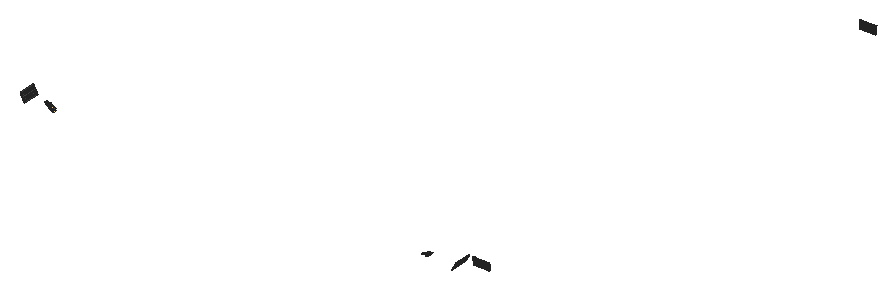
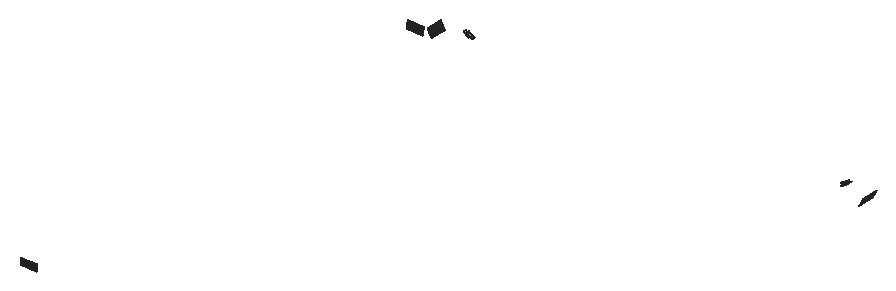
# SketchUp Ruby script. Lengths in inches.
U = 1.inch
M = Sketchup.active_model
def pt(a) = Geom::Point3d.new(a.map { |v| v * U })
def face(e, loops, mat)
  f = e.add_face(loops[0].map { |a| pt(a) })
  loops[1..].each { |l| e.add_face(l.map { |a| pt(a) }).erase! }
  f.material = f.back_material = mat if mat
  f
end
# faces: each face lists its corners as indices into pts; further lists are holes
def faces(e, pts, list, mat = nil) = list.each { |f| face(e, (f[0].is_a?(Array) ? f : [f]).map { |l| l.map { |i| pts[i] } }, mat) }
# xy, xz, yz: faces in a plane at the given z, y or x. An outline is a flat list of corners, or four numbers for a rectangle; further outlines are holes
def ring(l) = l.size == 4 ? [[l[0], l[1]], [l[2], l[1]], [l[2], l[3]], [l[0], l[3]]] : l.each_slice(2).to_a
def flat(e, list, mat, &to3) = list.each { |f| face(e, (f[0].is_a?(Array) ? f : [f]).map { |l| ring(l).map { |u, v| to3.(u, v) } }, mat) }
def xy(e, z, list, mat = nil) = flat(e, list, mat) { |x, y| [x, y, z] }
def xz(e, y, list, mat = nil) = flat(e, list, mat) { |x, z| [x, y, z] }
def yz(e, x, list, mat = nil) = flat(e, list, mat) { |y, z| [x, y, z] }
def lines(e, pts, list) = list.each { |a, b| e.add_line(pt(pts[a]), pt(pts[b])) }
# prism: a flat outline (further loops are holes) pulled along v
def prism(e, loops, v, mat = nil)
  f = face(e, loops, mat); d = Geom::Vector3d.new(v.map { |x| x * U })
  f.pushpull(f.normal.samedirection?(d) ? d.length : -d.length)
end
def box(e, o, s, mat = nil) = prism(e, [[o, [o[0] + s[0], o[1], o[2]], [o[0] + s[0], o[1] + s[1], o[2]], [o[0], o[1] + s[1], o[2]]]], [0, 0, s[2]], mat)
def at(x, y, z, deg = 0) = Geom::Transformation.translation(pt([x, y, z])) * Geom::Transformation.rotation(ORIGIN, Z_AXIS, deg.degrees)
def axes(o, x, y, z) = Geom::Transformation.new([*x, 0, *y, 0, *z, 0, *pt(o).to_a, 1])
def part(name) = M.definitions.add(name)
# library, detail: a bought-in or finely detailed component or shape, given as its bounding box
def library(name, o, s) = part(name).tap { |d| box(d.entities, o, s) }
def detail(e, o, s) = box(e.add_group.entities, o, s)
def put(e, d, t, mat = nil) = e.add_instance(d, t).tap { |i| i.material = mat if mat }
def group(e, t, mat = nil) = e.add_group.tap { |g| g.transformation = t; g.material = mat if mat }.entities
root = M.entities
M.materials.add("1432 AP 8245 TAR ROAD").color = [71, 72, 75]
M.materials.add("Outer Light").color = [251, 217, 152]
p = [[248.91,107.37,172.03],[249.07,107.37,171.79],[249.07,95.37,171.79],[248.91,95.37,172.03],[566.93,107.37,171.79],[567.09,107.37,172.03],
  [567.09,95.37,172.03],[566.93,95.37,171.79],[573,108.18,172.22],[573,108.24,171.9375],[585,108.24,171.9375],[585,108.18,172.22],
  [573,466.5,171.9375],[573,466.5625,172.22],[585,466.5625,172.22],[585,466.5,171.9375],[248.76,107.37,172.26],[248.76,95.37,172.26],
  [567.24,107.37,172.26],[567.24,95.37,172.26],[573,108.12,172.49],[585,108.12,172.49],[573,466.62,172.49],[585,466.62,172.49],
  [248.6,107.37,172.5],[248.6,95.37,172.5],[567.4,107.37,172.5],[567.4,95.37,172.5],[248.45,107.37,172.74],[248.45,95.37,172.74],
  [567.55,107.37,172.74],[567.55,95.37,172.74],[573,108.0625,172.77],[585,108.0625,172.77],[573,466.68,172.77],[585,466.68,172.77],
  [248.3,107.37,172.98],[248.3,95.37,172.98],[567.7,107.37,172.98],[567.7,95.37,172.98],[573,108.01,173.05],[585,108.01,173.05],
  [573,466.73,173.05],[585,466.73,173.05],[270.86,96.87,172.98],[271.01,96.87,172.91],[271.01,95.37,172.91],[270.86,95.37,172.98],
  [248.16,107.37,173.22],[248.16,95.37,173.22],[270.5625,96.87,173.11],[270.71,96.87,173.04],[270.71,95.37,173.04],[270.5625,95.37,173.11],
  [567.84,107.37,173.22],[567.84,95.37,173.22],[573,107.96,173.32],[585,107.96,173.32],[573,466.78,173.32],[585,466.78,173.32],
  [270.42,96.87,173.18],[270.42,95.37,173.18],[248.01,107.37,173.47],[248.01,95.37,173.47],[270.125,96.87,173.3125],[270.27,96.87,173.24],
  [270.27,95.37,173.24],[270.125,95.37,173.3125],[567.99,107.37,173.47],[567.99,95.37,173.47],[269.98,96.87,173.38],[269.98,95.37,173.38],
  [573,107.91,173.6],[585,107.91,173.6],[573,466.83,173.6],[585,466.83,173.6],[269.84,96.87,173.45],[269.84,95.37,173.45],
  [247.87,107.37,173.71],[247.87,95.37,173.71],[269.55,96.87,173.6],[269.69,96.87,173.53],[269.69,95.37,173.53],[269.55,95.37,173.6],
  [568.13,107.37,173.71],[568.13,95.37,173.71],[269.41,96.87,173.67],[269.41,95.37,173.67],[573,107.86,173.88],[585,107.86,173.88],
  [573,466.88,173.88],[585,466.88,173.88],[247.73,107.37,173.96],[247.73,95.37,173.96],[269.27,96.87,173.75],[269.27,95.37,173.75],
  [568.27,107.37,173.96],[568.27,95.37,173.96],[268.98,96.87,173.91],[269.125,96.87,173.83],[269.125,95.37,173.83],[268.98,95.37,173.91],
  [268.84,96.87,173.99],[268.84,95.37,173.99],[573,107.8125,174.16],[585,107.8125,174.16],[573,466.93,174.16],[585,466.93,174.16],
  [247.59,107.37,174.2],[247.59,95.37,174.2],[268.7,96.87,174.07],[268.7,95.37,174.07],[568.41,107.37,174.2],[568.41,95.37,174.2],
  [268.43,96.87,174.23],[268.56,96.87,174.15],[268.56,95.37,174.15],[268.43,95.37,174.23],[247.45,107.37,174.45],[247.45,95.37,174.45],
  [268.29,96.87,174.3125],[268.29,95.37,174.3125],[568.55,107.37,174.45],[568.55,95.37,174.45],[573,107.77,174.44],[585,107.77,174.44],
  [573,466.97,174.44],[585,466.97,174.44],[268.15,96.87,174.4],[268.15,95.37,174.4],[247.32,107.37,174.7],[247.32,95.37,174.7],
  [268.02,95.37,174.48],[268.15,95.37,174.4],[268.15,96.87,174.4],[268.02,96.87,174.48],[268.02,96.87,174.48],[268.02,95.37,174.48],
  [271.32,95.37,174.41],[271.18,95.37,174.48],[271.18,96.87,174.48],[271.32,96.87,174.41],[271.32,96.87,174.41],[271.18,96.87,174.48],
  [271.18,95.37,174.48],[271.32,95.37,174.41],[544.68,96.87,174.41],[544.55,96.87,174.35],[544.55,95.37,174.35],[544.68,95.37,174.41],
  [544.82,96.87,174.48],[544.82,95.37,174.48],[544.82,95.37,174.48],[544.68,95.37,174.41],[544.68,96.87,174.41],[544.82,96.87,174.48],
  [547.85,95.37,174.4],[547.98,95.37,174.48],[547.98,96.87,174.48],[547.85,96.87,174.4],[547.85,96.87,174.4],[547.98,96.87,174.48],
  [547.98,95.37,174.48],[547.85,95.37,174.4],[568.68,107.37,174.7],[568.68,95.37,174.7],[573,107.73,174.72],[585,107.73,174.72],
  [573,467.01,174.72],[585,467.01,174.72],[267.88,95.37,174.57],[267.88,96.87,174.57],[267.88,96.87,174.57],[267.88,95.37,174.57],
  [271.05,95.37,174.54],[270.91,95.37,174.6],[270.91,96.87,174.6],[271.05,96.87,174.54],[271.05,96.87,174.54],[270.91,96.87,174.6],
  [270.91,95.37,174.6],[271.05,95.37,174.54],[544.95,96.87,174.54],[544.95,95.37,174.54],[544.95,95.37,174.54],[544.95,96.87,174.54],
  [545.09,96.87,174.6],[545.09,95.37,174.6],[545.09,95.37,174.6],[545.09,96.87,174.6],[548.12,95.37,174.57],[548.12,96.87,174.57],
  [548.12,96.87,174.57],[548.12,95.37,174.57],[267.75,95.37,174.66],[267.75,96.87,174.66],[267.75,96.87,174.66],[267.75,95.37,174.66],
  [270.78,95.37,174.66],[270.78,96.87,174.66],[270.78,96.87,174.66],[270.78,95.37,174.66],[545.22,96.87,174.66],[545.22,95.37,174.66],
  [545.22,95.37,174.66],[545.22,96.87,174.66],[548.25,95.37,174.66],[548.25,96.87,174.66],[548.25,96.87,174.66],[548.25,95.37,174.66],
  [247.18,107.37,174.95],[247.18,95.37,174.95],[267.48,95.37,174.84],[267.61,95.37,174.75],[267.61,96.87,174.75],[267.48,96.87,174.84],
  [267.48,96.87,174.84],[267.61,96.87,174.75],[267.61,95.37,174.75],[267.48,95.37,174.84],[270.64,95.37,174.73],[270.51,95.37,174.8],
  [270.51,96.87,174.8],[270.64,96.87,174.73],[270.64,96.87,174.73],[270.51,96.87,174.8],[270.51,95.37,174.8],[270.64,95.37,174.73],
  [545.36,96.87,174.73],[545.36,95.37,174.73],[545.36,95.37,174.73],[545.36,96.87,174.73],[545.49,96.87,174.8],[545.49,95.37,174.8],
  [545.49,95.37,174.8],[545.49,96.87,174.8],[548.39,95.37,174.75],[548.39,96.87,174.75],[548.39,96.87,174.75],[548.39,95.37,174.75],
  [548.52,95.37,174.84],[548.52,96.87,174.84],[548.52,96.87,174.84],[548.52,95.37,174.84],[568.82,107.37,174.95],[568.82,95.37,174.95],
  [573,107.69,175],[585,107.69,175],[573,467.05,175],[585,467.05,175],[267.34,95.37,174.93],[267.34,96.87,174.93],
  [267.34,96.87,174.93],[267.34,95.37,174.93],[270.375,95.37,174.86],[270.375,96.87,174.86],[270.375,96.87,174.86],[270.375,95.37,174.86],
  [545.625,96.87,174.86],[545.625,95.37,174.86],[545.625,95.37,174.86],[545.625,96.87,174.86],[548.66,95.37,174.93],[548.66,96.87,174.93],
  [548.66,96.87,174.93],[548.66,95.37,174.93],[247.05,107.37,175.2],[247.05,95.37,175.2],[267.21,95.37,175.02],[267.21,96.87,175.02],
  [267.21,96.87,175.02],[267.21,95.37,175.02],[270.24,95.37,174.93],[270.11,95.37,175],[270.11,96.87,175],[270.24,96.87,174.93],
  [270.24,96.87,174.93],[270.11,96.87,175],[270.11,95.37,175],[270.24,95.37,174.93],[545.76,96.87,174.93],[545.76,95.37,174.93],
  [545.76,95.37,174.93],[545.76,96.87,174.93],[545.89,96.87,175],[545.89,95.37,175],[545.89,95.37,175],[545.89,96.87,175],
  [548.79,95.37,175.02],[548.79,96.87,175.02],[548.79,96.87,175.02],[548.79,95.37,175.02],[568.95,107.37,175.2],[568.95,95.37,175.2],
  [267.08,95.37,175.11],[267.08,96.87,175.11],[267.08,96.87,175.11],[267.08,95.37,175.11],[269.98,95.37,175.07],[269.98,96.87,175.07],
  [269.98,96.87,175.07],[269.98,95.37,175.07],[546.02,96.87,175.07],[546.02,95.37,175.07],[546.02,95.37,175.07],[546.02,96.87,175.07],
  [548.92,95.37,175.11],[548.92,96.87,175.11],[548.92,96.87,175.11],[548.92,95.37,175.11],[573,107.65,175.28],[585,107.65,175.28],
  [573,467.09,175.28],[585,467.09,175.28],[266.95,95.37,175.21],[266.95,96.87,175.21],[266.95,96.87,175.21],[266.95,95.37,175.21],
  [269.85,95.37,175.14],[269.72,95.37,175.21],[269.72,96.87,175.21],[269.85,96.87,175.14],[269.85,96.87,175.14],[269.72,96.87,175.21],
  [269.72,95.37,175.21],[269.85,95.37,175.14],[546.15,96.87,175.14],[546.15,95.37,175.14],[546.15,95.37,175.14],[546.15,96.87,175.14],
  [546.28,96.87,175.21],[546.28,95.37,175.21],[546.28,95.37,175.21],[546.28,96.87,175.21],[549.05,95.37,175.21],[549.05,96.87,175.21],
  [549.05,96.87,175.21],[549.05,95.37,175.21],[246.92,107.37,175.45],[246.92,95.37,175.45],[266.82,95.37,175.3],[266.82,96.87,175.3],
  [266.82,96.87,175.3],[266.82,95.37,175.3],[269.59,95.37,175.29],[269.59,96.87,175.29],[269.59,96.87,175.29],[269.59,95.37,175.29],
  [546.41,96.87,175.29],[546.41,95.37,175.29],[546.41,95.37,175.29],[546.41,96.87,175.29],[549.18,95.37,175.3],[549.18,96.87,175.3],
  [549.18,96.87,175.3],[549.18,95.37,175.3],[569.08,107.37,175.45],[569.08,95.37,175.45],[266.69,95.37,175.4],[266.69,96.87,175.4],
  [266.69,96.87,175.4],[266.69,95.37,175.4],[269.46,95.37,175.36],[269.46,96.87,175.36],[269.46,96.87,175.36],[269.46,95.37,175.36],
  [546.54,96.87,175.36],[546.54,95.37,175.36],[546.54,95.37,175.36],[546.54,96.87,175.36],[549.31,95.37,175.4],[549.31,96.87,175.4],
  [549.31,96.87,175.4],[549.31,95.37,175.4],[573,107.62,175.5625],[585,107.62,175.5625],[573,467.12,175.5625],[585,467.12,175.5625],
  [246.8,107.37,175.7],[246.8,95.37,175.7],[266.5625,95.37,175.5],[266.5625,96.87,175.5],[266.5625,96.87,175.5],[266.5625,95.37,175.5],
  [269.33,95.37,175.4375],[269.2,95.37,175.51],[269.2,96.87,175.51],[269.33,96.87,175.4375],[269.33,96.87,175.4375],[269.2,96.87,175.51],
  [269.2,95.37,175.51],[269.33,95.37,175.4375],[546.67,96.87,175.4375],[546.67,95.37,175.4375],[546.67,95.37,175.4375],[546.67,96.87,175.4375],
  [546.8,96.87,175.51],[546.8,95.37,175.51],[546.8,95.37,175.51],[546.8,96.87,175.51],[549.4375,95.37,175.5],[549.4375,96.87,175.5],
  [549.4375,96.87,175.5],[549.4375,95.37,175.5],[569.2,107.37,175.7],[569.2,95.37,175.7],[266.44,95.37,175.59],[266.44,96.87,175.59],
  [266.44,96.87,175.59],[266.44,95.37,175.59],[269.07,95.37,175.59],[269.07,96.87,175.59],[269.07,96.87,175.59],[269.07,95.37,175.59],
  [546.93,96.87,175.59],[546.93,95.37,175.59],[546.93,95.37,175.59],[546.93,96.87,175.59],[549.56,95.37,175.59],[549.56,96.87,175.59],
  [549.56,96.87,175.59],[549.56,95.37,175.59],[266.31,95.37,175.69],[266.31,96.87,175.69],[266.31,96.87,175.69],[266.31,95.37,175.69],
  [268.95,95.37,175.67],[268.95,96.87,175.67],[268.95,96.87,175.67],[268.95,95.37,175.67],[547.05,96.87,175.67],[547.05,95.37,175.67],
  [547.05,95.37,175.67],[547.05,96.87,175.67],[549.69,95.37,175.69],[549.69,96.87,175.69],[549.69,96.87,175.69],[549.69,95.37,175.69],
  [573,107.59,175.84],[585,107.59,175.84],[573,467.15,175.84],[585,467.15,175.84],[246.67,107.37,175.95],[246.67,95.37,175.95],
  [266.18,95.37,175.79],[266.18,96.87,175.79],[266.18,96.87,175.79],[266.18,95.37,175.79],[268.82,95.37,175.75],[268.69,95.37,175.83],
  [268.69,96.87,175.83],[268.82,96.87,175.75],[268.82,96.87,175.75],[268.69,96.87,175.83],[268.69,95.37,175.83],[268.82,95.37,175.75],
  [547.18,96.87,175.75],[547.18,95.37,175.75],[547.18,95.37,175.75],[547.18,96.87,175.75],[547.31,96.87,175.83],[547.31,95.37,175.83],
  [547.31,95.37,175.83],[547.31,96.87,175.83],[549.82,95.37,175.79],[549.82,96.87,175.79],[549.82,96.87,175.79],[549.82,95.37,175.79],
  [569.33,107.37,175.95],[569.33,95.37,175.95],[266.06,95.37,175.89],[266.06,96.87,175.89],[266.06,96.87,175.89],[266.06,95.37,175.89],
  [268.57,95.37,175.91],[268.57,96.87,175.91],[268.57,96.87,175.91],[268.57,95.37,175.91],[547.43,96.87,175.91],[547.43,95.37,175.91],
  [547.43,95.37,175.91],[547.43,96.87,175.91],[549.94,95.37,175.89],[549.94,96.87,175.89],[549.94,96.87,175.89],[549.94,95.37,175.89],
  [573,107.56,176.12],[585,107.56,176.12],[573,467.18,176.12],[585,467.18,176.12],[265.93,95.37,176],[265.93,96.87,176],
  [265.93,96.87,176],[265.93,95.37,176],[268.44,95.37,175.99],[268.44,96.87,175.99],[268.44,96.87,175.99],[268.44,95.37,175.99],
  [547.56,96.87,175.99],[547.56,95.37,175.99],[547.56,95.37,175.99],[547.56,96.87,175.99],[550.07,95.37,176],[550.07,96.87,176],
  [550.07,96.87,176],[550.07,95.37,176],[246.55,107.37,176.21],[246.55,95.37,176.21],[265.81,95.37,176.1],[265.81,96.87,176.1],
  [265.81,96.87,176.1],[265.81,95.37,176.1],[268.32,95.37,176.08],[268.32,96.87,176.08],[268.32,96.87,176.08],[268.32,95.37,176.08],
  [547.68,96.87,176.08],[547.68,95.37,176.08],[547.68,95.37,176.08],[547.68,96.87,176.08],[550.19,95.37,176.1],[550.19,96.87,176.1],
  [550.19,96.87,176.1],[550.19,95.37,176.1],[569.45,107.37,176.21],[569.45,95.37,176.21],[265.6875,95.37,176.2],[265.6875,96.87,176.2],
  [265.6875,96.87,176.2],[265.6875,95.37,176.2],[268.2,95.37,176.16],[268.2,96.87,176.16],[268.2,96.87,176.16],[268.2,95.37,176.16],
  [547.8,96.87,176.16],[547.8,95.37,176.16],[547.8,95.37,176.16],[547.8,96.87,176.16],[550.3125,95.37,176.2],[550.3125,96.87,176.2],
  [550.3125,96.87,176.2],[550.3125,95.37,176.2],[573,107.53,176.4],[585,107.53,176.4],[573,467.21,176.4],[585,467.21,176.4],
  [246.43,107.37,176.46],[246.43,95.37,176.46],[265.5625,95.37,176.31],[265.5625,96.87,176.31],[265.5625,96.87,176.31],[265.5625,95.37,176.31],
  [268.07,95.37,176.25],[267.95,95.37,176.33],[267.95,96.87,176.33],[268.07,96.87,176.25],[268.07,96.87,176.25],[267.95,96.87,176.33],
  [267.95,95.37,176.33],[268.07,95.37,176.25],[547.93,96.87,176.25],[547.93,95.37,176.25],[547.93,95.37,176.25],[547.93,96.87,176.25],
  [548.05,96.87,176.33],[548.05,95.37,176.33],[548.05,95.37,176.33],[548.05,96.87,176.33],[550.4375,95.37,176.31],[550.4375,96.87,176.31],
  [550.4375,96.87,176.31],[550.4375,95.37,176.31],[569.57,107.37,176.46],[569.57,95.37,176.46],[265.44,95.37,176.41],[265.44,96.87,176.41],
  [265.44,96.87,176.41],[265.44,95.37,176.41],[267.83,95.37,176.42],[267.83,96.87,176.42],[267.83,96.87,176.42],[267.83,95.37,176.42],
  [548.17,96.87,176.42],[548.17,95.37,176.42],[548.17,95.37,176.42],[548.17,96.87,176.42],[550.56,95.37,176.41],[550.56,96.87,176.41],
  [550.56,96.87,176.41],[550.56,95.37,176.41],[265.32,95.37,176.52],[265.32,96.87,176.52],[265.32,96.87,176.52],[265.32,95.37,176.52],
  [267.71,95.37,176.51],[267.71,96.87,176.51],[267.71,96.87,176.51],[267.71,95.37,176.51],[548.29,96.87,176.51],[548.29,95.37,176.51],
  [548.29,95.37,176.51],[548.29,96.87,176.51],[550.68,95.37,176.52],[550.68,96.87,176.52],[550.68,96.87,176.52],[550.68,95.37,176.52],
  [573,107.5,176.6875],[585,107.5,176.6875],[573,467.24,176.6875],[585,467.24,176.6875],[246.31,107.37,176.72],[246.31,95.37,176.72],
  [265.2,95.37,176.63],[265.2,96.87,176.63],[265.2,96.87,176.63],[265.2,95.37,176.63],[267.59,95.37,176.6],[267.59,96.87,176.6],
  [267.59,96.87,176.6],[267.59,95.37,176.6],[548.41,96.87,176.6],[548.41,95.37,176.6],[548.41,95.37,176.6],[548.41,96.87,176.6],
  [550.8,95.37,176.63],[550.8,96.87,176.63],[550.8,96.87,176.63],[550.8,95.37,176.63],[569.69,107.37,176.72],[569.69,95.37,176.72],
  [265.08,95.37,176.74],[265.08,96.87,176.74],[265.08,96.87,176.74],[265.08,95.37,176.74],[267.47,95.37,176.6875],[267.47,96.87,176.6875],
  [267.47,96.87,176.6875],[267.47,95.37,176.6875],[548.53,96.87,176.6875],[548.53,95.37,176.6875],[548.53,95.37,176.6875],[548.53,96.87,176.6875],
  [550.92,95.37,176.74],[550.92,96.87,176.74],[550.92,96.87,176.74],[550.92,95.37,176.74],[246.1875,107.37,176.98],[246.1875,95.37,176.98],
  [264.97,95.37,176.85],[264.97,96.87,176.85],[264.97,96.87,176.85],[264.97,95.37,176.85],[267.35,95.37,176.78],[267.35,96.87,176.78],
  [267.35,96.87,176.78],[267.35,95.37,176.78],[548.65,96.87,176.78],[548.65,95.37,176.78],[548.65,95.37,176.78],[548.65,96.87,176.78],
  [551.03,95.37,176.85],[551.03,96.87,176.85],[551.03,96.87,176.85],[551.03,95.37,176.85],[569.8125,107.37,176.98],[569.8125,95.37,176.98],
  [573,107.48,176.97],[585,107.48,176.97],[573,467.26,176.97],[585,467.26,176.97],[264.85,95.37,176.96],[264.85,96.87,176.96],
  [264.85,96.87,176.96],[264.85,95.37,176.96],[267.24,95.37,176.87],[267.24,96.87,176.87],[267.24,96.87,176.87],[267.24,95.37,176.87],
  [548.76,96.87,176.87],[548.76,95.37,176.87],[548.76,95.37,176.87],[548.76,96.87,176.87],[551.15,95.37,176.96],[551.15,96.87,176.96],
  [551.15,96.87,176.96],[551.15,95.37,176.96],[267.12,95.37,176.96],[267.12,96.87,176.96],[267.12,96.87,176.96],[267.12,95.37,176.96],
  [548.88,96.87,176.96],[548.88,95.37,176.96],[548.88,95.37,176.96],[548.88,96.87,176.96],[246.07,107.37,177.24],[246.07,95.37,177.24],
  [264.73,95.37,177.07],[264.73,96.87,177.07],[264.73,96.87,177.07],[264.73,95.37,177.07],[267,95.37,177.06],[267,96.87,177.06],
  [267,96.87,177.06],[267,95.37,177.06],[549,96.87,177.06],[549,95.37,177.06],[549,95.37,177.06],[549,96.87,177.06],
  [551.27,95.37,177.07],[551.27,96.87,177.07],[551.27,96.87,177.07],[551.27,95.37,177.07],[569.93,107.37,177.24],[569.93,95.37,177.24],
  [573,107.46,177.25],[585,107.46,177.25],[573,467.28,177.25],[585,467.28,177.25],[264.62,95.37,177.18],[264.62,96.87,177.18],
  [264.62,96.87,177.18],[264.62,95.37,177.18],[266.89,95.37,177.15],[266.89,96.87,177.15],[266.89,96.87,177.15],[266.89,95.37,177.15],
  [549.11,96.87,177.15],[549.11,95.37,177.15],[549.11,95.37,177.15],[549.11,96.87,177.15],[551.38,95.37,177.18],[551.38,96.87,177.18],
  [551.38,96.87,177.18],[551.38,95.37,177.18],[245.96,107.37,177.49],[245.96,95.37,177.49],[264.5,95.37,177.3],[264.5,96.87,177.3],
  [264.5,96.87,177.3],[264.5,95.37,177.3],[266.77,95.37,177.25],[266.66,95.37,177.34],[266.66,96.87,177.34],[266.77,96.87,177.25],
  [266.77,96.87,177.25],[266.66,96.87,177.34],[266.66,95.37,177.34],[266.77,95.37,177.25],[549.23,96.87,177.25],[549.23,95.37,177.25],
  [549.23,95.37,177.25],[549.23,96.87,177.25],[549.34,96.87,177.34],[549.34,95.37,177.34],[549.34,95.37,177.34],[549.34,96.87,177.34],
  [551.5,95.37,177.3],[551.5,96.87,177.3],[551.5,96.87,177.3],[551.5,95.37,177.3],[570.04,107.37,177.49],[570.04,95.37,177.49],
  [573,107.44,177.53],[585,107.44,177.53]]
faces(root,p,[[0,1,2,3],[4,5,6,7],[8,9,10,11],[12,13,14,15],[16,0,3,17],[5,18,19,6],[20,8,11,21],[13,22,23,14],
  [24,16,17,25],[18,26,27,19],[28,24,25,29],[26,30,31,27],[32,20,21,33],[22,34,35,23],[36,28,29,37],[30,38,39,31],
  [40,32,33,41],[34,42,43,35],[48,36,37,49],[38,54,55,39],[56,40,41,57],[42,58,59,43],[62,48,49,63],[54,68,69,55],
  [72,56,57,73],[58,74,75,59],[78,62,63,79],[68,84,85,69],[88,72,73,89],[74,90,91,75],[92,78,79,93],[84,96,97,85],
  [104,88,89,105],[90,106,107,91],[108,92,93,109],[96,112,113,97],[118,108,109,119],[112,122,123,113],[124,104,105,125],[106,126,127,107],
  [130,118,119,131],[132,133,134,135],[138,139,140,141],[152,153,154,155],[156,157,158,159],[122,164,165,123],[166,124,125,167],[126,168,169,127],
  [170,132,135,171],[174,175,176,177],[139,174,177,140],[184,152,155,185],[188,184,185,189],[157,190,191,158],[194,170,171,195],[175,198,199,176],
  [204,188,189,205],[190,206,207,191],[210,130,131,211],[212,213,214,215],[213,194,195,214],[220,221,222,223],[198,220,223,199],[230,204,205,231],
  [234,230,231,235],[206,236,237,207],[236,240,241,237],[164,244,245,165],[246,166,167,247],[168,248,249,169],[250,212,215,251],[221,254,255,222],
  [260,234,235,261],[240,262,263,241],[266,210,211,267],[268,250,251,269],[272,273,274,275],[254,272,275,255],[282,260,261,283],[286,282,283,287],
  [262,288,289,263],[244,292,293,245],[294,268,269,295],[273,298,299,274],[304,286,287,305],[288,306,307,289],[310,246,247,311],[248,312,313,249],
  [314,294,295,315],[318,319,320,321],[298,318,321,299],[328,304,305,329],[332,328,329,333],[306,334,335,307],[338,266,267,339],[340,314,315,341],
  [319,344,345,320],[350,332,333,351],[334,352,353,335],[292,356,357,293],[358,340,341,359],[344,362,363,345],[368,350,351,369],[352,370,371,353],
  [374,310,311,375],[312,376,377,313],[378,338,339,379],[380,358,359,381],[384,385,386,387],[362,384,387,363],[394,368,369,395],[398,394,395,399],
  [370,400,401,371],[356,404,405,357],[406,380,381,407],[385,410,411,386],[416,398,399,417],[400,418,419,401],[422,406,407,423],[410,426,427,411],
  [432,416,417,433],[418,434,435,419],[438,374,375,439],[376,440,441,377],[442,378,379,443],[444,422,423,445],[448,449,450,451],[426,448,451,427],
  [458,432,433,459],[462,458,459,463],[434,464,465,435],[404,468,469,405],[470,444,445,471],[449,474,475,450],[480,462,463,481],[464,482,483,465],
  [486,438,439,487],[440,488,489,441],[490,470,471,491],[474,494,495,475],[500,480,481,501],[482,502,503,483],[506,442,443,507],[508,490,491,509],
  [494,512,513,495],[518,500,501,519],[502,520,521,503],[468,524,525,469],[526,508,509,527],[512,530,531,513],[536,518,519,537],[520,538,539,521],
  [542,486,487,543],[488,544,545,489],[546,506,507,547],[548,526,527,549],[552,553,554,555],[530,552,555,531],[562,536,537,563],[566,562,563,567],
  [538,568,569,539],[524,572,573,525],[574,548,549,575],[553,578,579,554],[584,566,567,585],[568,586,587,569],[590,574,575,591],[578,594,595,579],
  [600,584,585,601],[586,602,603,587],[606,542,543,607],[544,608,609,545],[610,546,547,611],[612,590,591,613],[594,616,617,595],[622,600,601,623],
  [602,624,625,603],[572,628,629,573],[630,612,613,631],[616,634,635,617],[640,622,623,641],[624,642,643,625],[646,610,611,647],[648,630,631,649],
  [634,652,653,635],[658,640,641,659],[642,660,661,643],[628,664,665,629],[666,606,607,667],[608,668,669,609],[670,648,649,671],[652,674,675,653],
  [680,658,659,681],[660,682,683,661],[674,686,687,675],[692,680,681,693],[694,646,647,695],[696,670,671,697],[686,700,701,687],[706,692,693,707],
  [682,708,709,683],[664,712,713,665],[714,666,667,715],[668,716,717,669],[718,696,697,719],[700,722,723,701],[728,706,707,729],[708,730,731,709],
  [734,694,695,735],[736,718,719,737],[740,741,742,743],[722,740,743,723],[750,728,729,751],[754,750,751,755],[730,756,757,731],[712,760,761,713],
  [762,714,715,763]],"1432 AP 8245 TAR ROAD")
faces(root,p,[[44,45,46,47],[50,51,52,53],[51,44,47,52],[60,50,53,61],[64,65,66,67],[65,60,61,66],[70,64,67,71],[76,70,71,77],
  [80,81,82,83],[81,76,77,82],[86,80,83,87],[94,86,87,95],[98,99,100,101],[99,94,95,100],[102,98,101,103],[110,102,103,111],
  [114,115,116,117],[115,110,111,116],[120,114,117,121],[128,120,121,129],[136,128,129,137],[142,143,144,145],[146,147,148,149],[150,146,149,151],
  [160,161,162,163],[172,136,137,173],[178,179,180,181],[143,178,181,144],[182,150,151,183],[186,182,183,187],[161,192,193,162],[196,172,173,197],
  [179,200,201,180],[202,186,187,203],[192,208,209,193],[216,217,218,219],[217,196,197,218],[224,225,226,227],[200,224,227,201],[228,202,203,229],
  [232,228,229,233],[208,238,239,209],[238,242,243,239],[252,216,219,253],[225,256,257,226],[258,232,233,259],[242,264,265,243],[270,252,253,271],
  [276,277,278,279],[256,276,279,257],[280,258,259,281],[284,280,281,285],[264,290,291,265],[296,270,271,297],[277,300,301,278],[302,284,285,303],
  [290,308,309,291],[316,296,297,317],[322,323,324,325],[300,322,325,301],[326,302,303,327],[330,326,327,331],[308,336,337,309],[342,316,317,343],
  [323,346,347,324],[348,330,331,349],[336,354,355,337],[360,342,343,361],[346,364,365,347],[366,348,349,367],[354,372,373,355],[382,360,361,383],
  [388,389,390,391],[364,388,391,365],[392,366,367,393],[396,392,393,397],[372,402,403,373],[408,382,383,409],[389,412,413,390],[414,396,397,415],
  [402,420,421,403],[424,408,409,425],[412,428,429,413],[430,414,415,431],[420,436,437,421],[446,424,425,447],[452,453,454,455],[428,452,455,429],
  [456,430,431,457],[460,456,457,461],[436,466,467,437],[472,446,447,473],[453,476,477,454],[478,460,461,479],[466,484,485,467],[492,472,473,493],
  [476,496,497,477],[498,478,479,499],[484,504,505,485],[510,492,493,511],[496,514,515,497],[516,498,499,517],[504,522,523,505],[528,510,511,529],
  [514,532,533,515],[534,516,517,535],[522,540,541,523],[550,528,529,551],[556,557,558,559],[532,556,559,533],[560,534,535,561],[564,560,561,565],
  [540,570,571,541],[576,550,551,577],[557,580,581,558],[582,564,565,583],[570,588,589,571],[592,576,577,593],[580,596,597,581],[598,582,583,599],
  [588,604,605,589],[614,592,593,615],[596,618,619,597],[620,598,599,621],[604,626,627,605],[632,614,615,633],[618,636,637,619],[638,620,621,639],
  [626,644,645,627],[650,632,633,651],[636,654,655,637],[656,638,639,657],[644,662,663,645],[672,650,651,673],[654,676,677,655],[678,656,657,679],
  [662,684,685,663],[676,688,689,677],[690,678,679,691],[698,672,673,699],[688,702,703,689],[704,690,691,705],[684,710,711,685],[720,698,699,721],
  [702,724,725,703],[726,704,705,727],[710,732,733,711],[738,720,721,739],[744,745,746,747],[724,744,747,725],[748,726,727,749],[752,748,749,753],
  [732,758,759,733]],"Outer Light")
